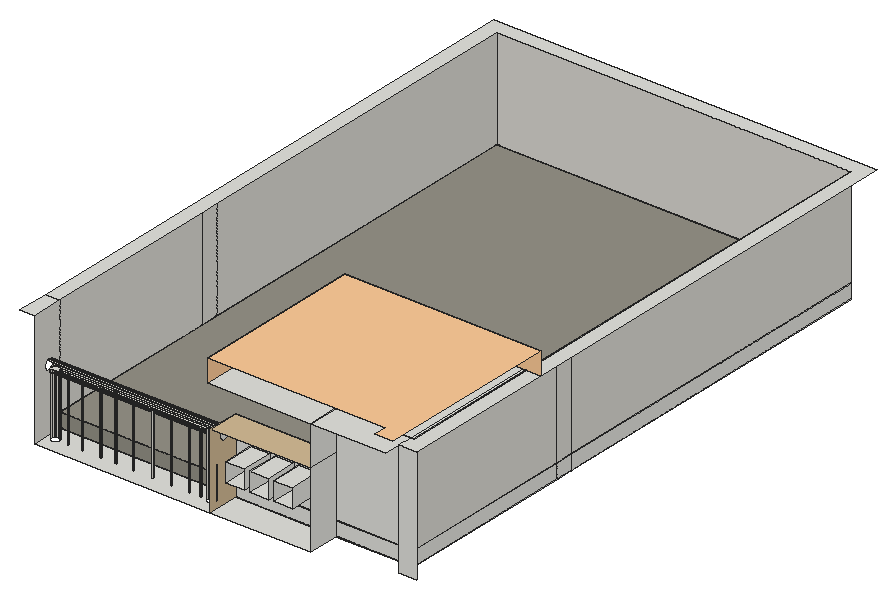
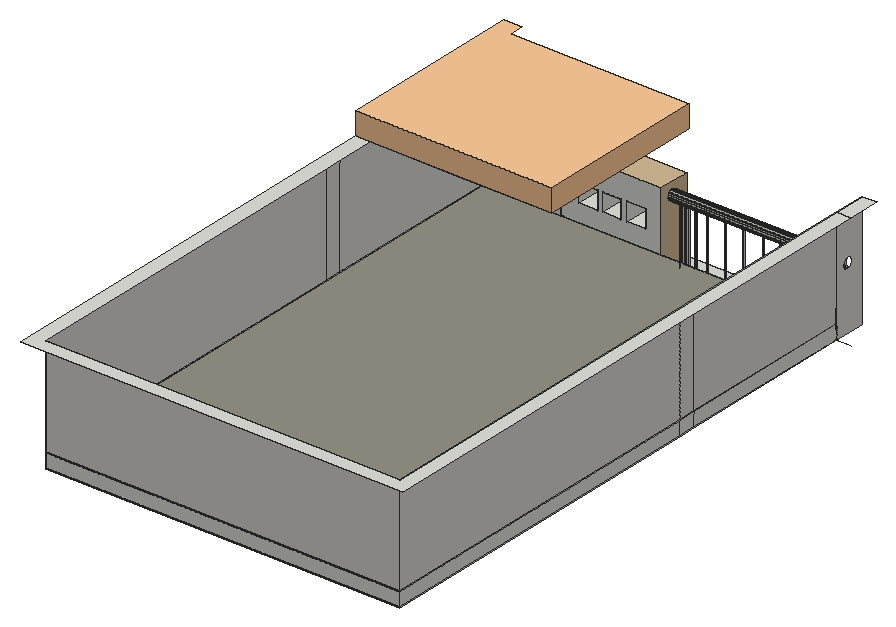
# SketchUp Ruby script. Lengths in inches.
U = 1.inch
M = Sketchup.active_model
def pt(a) = Geom::Point3d.new(a.map { |v| v * U })
def face(e, loops, mat)
  f = e.add_face(loops[0].map { |a| pt(a) })
  loops[1..].each { |l| e.add_face(l.map { |a| pt(a) }).erase! }
  f.material = f.back_material = mat if mat
  f
end
# faces: each face lists its corners as indices into pts; further lists are holes
def faces(e, pts, list, mat = nil) = list.each { |f| face(e, (f[0].is_a?(Array) ? f : [f]).map { |l| l.map { |i| pts[i] } }, mat) }
# xy, xz, yz: faces in a plane at the given z, y or x. An outline is a flat list of corners, or four numbers for a rectangle; further outlines are holes
def ring(l) = l.size == 4 ? [[l[0], l[1]], [l[2], l[1]], [l[2], l[3]], [l[0], l[3]]] : l.each_slice(2).to_a
def flat(e, list, mat, &to3) = list.each { |f| face(e, (f[0].is_a?(Array) ? f : [f]).map { |l| ring(l).map { |u, v| to3.(u, v) } }, mat) }
def xy(e, z, list, mat = nil) = flat(e, list, mat) { |x, y| [x, y, z] }
def xz(e, y, list, mat = nil) = flat(e, list, mat) { |x, z| [x, y, z] }
def yz(e, x, list, mat = nil) = flat(e, list, mat) { |y, z| [x, y, z] }
def lines(e, pts, list) = list.each { |a, b| e.add_line(pt(pts[a]), pt(pts[b])) }
# prism: a flat outline (further loops are holes) pulled along v
def prism(e, loops, v, mat = nil)
  f = face(e, loops, mat); d = Geom::Vector3d.new(v.map { |x| x * U })
  f.pushpull(f.normal.samedirection?(d) ? d.length : -d.length)
end
def box(e, o, s, mat = nil) = prism(e, [[o, [o[0] + s[0], o[1], o[2]], [o[0] + s[0], o[1] + s[1], o[2]], [o[0], o[1] + s[1], o[2]]]], [0, 0, s[2]], mat)
def at(x, y, z, deg = 0) = Geom::Transformation.translation(pt([x, y, z])) * Geom::Transformation.rotation(ORIGIN, Z_AXIS, deg.degrees)
def axes(o, x, y, z) = Geom::Transformation.new([*x, 0, *y, 0, *z, 0, *pt(o).to_a, 1])
def part(name) = M.definitions.add(name)
# library, detail: a bought-in or finely detailed component or shape, given as its bounding box
def library(name, o, s) = part(name).tap { |d| box(d.entities, o, s) }
def detail(e, o, s) = box(e.add_group.entities, o, s)
def put(e, d, t, mat = nil) = e.add_instance(d, t).tap { |i| i.material = mat if mat }
def group(e, t, mat = nil) = e.add_group.tap { |g| g.transformation = t; g.material = mat if mat }.entities
root = M.entities
M.materials.add("[Color C02]").color = [255, 204, 153]
M.materials.add("[Formica Beige]").color = [211, 187, 149]
M.materials.add("[Formica Graystone]").color = [149, 146, 135]
M.materials.add("[Terrazzo Tile Light]").color = [219, 217, 210]
xy(root,120,[[[9,41.58,119.1,61.39],[14.33,48.46,13.65,48.55,13.02,48.81,12.48,49.23,12.06,49.77,11.8,50.4,11.71,51.08,11.8,51.76,12.06,52.4,12.48,52.9375,13.02,53.36,13.65,53.62,14.33,53.71,15.01,53.62,15.64,53.36,16.1875,52.9375,16.6,52.4,16.87,51.76,16.96,51.08,16.87,50.4,16.6,49.77,16.1875,49.23,15.64,48.81,15.01,48.55],[112.21,48.46,111.53,48.55,110.89,48.81,110.35,49.23,109.93,49.77,109.67,50.4,109.58,51.08,109.67,51.76,109.93,52.4,110.35,52.9375,110.89,53.36,111.53,53.62,112.21,53.71,112.89,53.62,113.52,53.36,114.0625,52.9375,114.48,52.4,114.74,51.76,114.83,51.08,114.74,50.4,114.48,49.77,114.0625,49.23,113.52,48.81,112.89,48.55],[75.6,50.32,75.46,50.34,75.32,50.4,75.21,50.48,75.12,50.6,75.0625,50.74,75.04,50.88,75.0625,51.03,75.12,51.16,75.21,51.28,75.32,51.37,75.46,51.43,75.6,51.44,75.75,51.43,75.89,51.37,76,51.28,76.09,51.16,76.15,51.03,76.17,50.88,76.15,50.74,76.09,50.6,76,50.48,75.89,50.4,75.75,50.34],[31.29,50.32,31.15,50.34,31.01,50.4,30.89,50.48,30.8,50.6,30.75,50.74,30.73,50.88,30.75,51.03,30.8,51.16,30.89,51.28,31.01,51.37,31.15,51.43,31.29,51.44,31.4375,51.43,31.57,51.37,31.69,51.28,31.78,51.16,31.84,51.03,31.85,50.88,31.84,50.74,31.78,50.6,31.69,50.48,31.57,50.4,31.4375,50.34],[52.1,50.32,51.96,50.34,51.82,50.4,51.71,50.48,51.62,50.6,51.5625,50.74,51.54,50.88,51.5625,51.03,51.62,51.16,51.71,51.28,51.82,51.37,51.96,51.43,52.1,51.44,52.25,51.43,52.39,51.37,52.5,51.28,52.59,51.16,52.65,51.03,52.67,50.88,52.65,50.74,52.59,50.6,52.5,50.48,52.39,50.4,52.25,50.34],[63.23,50.32,63.08,50.34,62.95,50.4,62.83,50.48,62.74,50.6,62.6875,50.74,62.67,50.88,62.6875,51.03,62.74,51.16,62.83,51.28,62.95,51.37,63.08,51.43,63.23,51.44,63.375,51.43,63.51,51.37,63.63,51.28,63.72,51.16,63.77,51.03,63.79,50.88,63.77,50.74,63.72,50.6,63.63,50.48,63.51,50.4,63.375,50.34],[42.67,50.32,42.52,50.34,42.39,50.4,42.27,50.48,42.18,50.6,42.125,50.74,42.1,50.88,42.125,51.03,42.18,51.16,42.27,51.28,42.39,51.37,42.52,51.43,42.67,51.44,42.8125,51.43,42.95,51.37,43.06,51.28,43.15,51.16,43.21,51.03,43.23,50.88,43.21,50.74,43.15,50.6,43.06,50.48,42.95,50.4,42.8125,50.34],[87.1,50.32,86.96,50.34,86.82,50.4,86.71,50.48,86.62,50.6,86.5625,50.74,86.54,50.88,86.5625,51.03,86.62,51.16,86.71,51.28,86.82,51.37,86.96,51.43,87.1,51.44,87.25,51.43,87.39,51.37,87.5,51.28,87.59,51.16,87.65,51.03,87.67,50.88,87.65,50.74,87.59,50.6,87.5,50.48,87.39,50.4,87.25,50.34],[22.54,50.32,22.4,50.34,22.26,50.4,22.14,50.48,22.05,50.6,22,50.74,21.98,50.88,22,51.03,22.05,51.16,22.14,51.28,22.26,51.37,22.4,51.43,22.54,51.44,22.6875,51.43,22.82,51.37,22.94,51.28,23.03,51.16,23.09,51.03,23.1,50.88,23.09,50.74,23.03,50.6,22.94,50.48,22.82,50.4,22.6875,50.34],[105.42,50.32,105.27,50.34,105.14,50.4,105.02,50.48,104.93,50.6,104.875,50.74,104.85,50.88,104.875,51.03,104.93,51.16,105.02,51.28,105.14,51.37,105.27,51.43,105.42,51.44,105.5625,51.43,105.7,51.37,105.81,51.28,105.9,51.16,105.96,51.03,105.98,50.88,105.96,50.74,105.9,50.6,105.81,50.48,105.7,50.4,105.5625,50.34],[98.42,50.32,98.27,50.34,98.14,50.4,98.02,50.48,97.93,50.6,97.875,50.74,97.85,50.88,97.875,51.03,97.93,51.16,98.02,51.28,98.14,51.37,98.27,51.43,98.42,51.44,98.5625,51.43,98.7,51.37,98.81,51.28,98.9,51.16,98.96,51.03,98.98,50.88,98.96,50.74,98.9,50.6,98.81,50.48,98.7,50.4,98.5625,50.34]],[119.1,41.58,181.98,61.39],[9,61.39,231,172.96],[9,172.96,231,184.44],[9,184.44,231,403.39]])
xy(root,120.27,[[9,61.39,231,403.39]])
xy(root,129,[[9,61.39,231,403.39]])
xy(root,129.27,[[9,61.39,231,403.39]],"[Formica Graystone]")
xy(root,140.26,[[128.8125,41.58,140.5625,61.39],[144.125,41.58,155.875,61.39],[158.8125,41.58,170.5625,61.39]])
xy(root,152.01,[[128.8125,41.58,140.5625,61.39],[144.125,41.58,155.875,61.39],[158.8125,41.58,170.5625,61.39]])
xy(root,159.78,[[12.24,49.53,16.42,49.53,16.6,49.77,16.87,50.4,16.96,51.08,16.87,51.76,16.6,52.4,16.1875,52.9375,15.64,53.36,15.01,53.62,14.33,53.71,13.65,53.62,13.02,53.36,12.48,52.9375,12.06,52.4,11.8,51.76,11.71,51.08,11.8,50.4,12.06,49.77]])
xy(root,166.92,[[119.1,41.58,181.98,61.39]],"[Formica Beige]")
xy(root,192,[[0,41.58,9,61.39],[117.3125,41.58,181.98,149.14],[181.98,41.58,228.875,61.39],[228.875,52.39,240,52.39,240,149.14,231,149.14,231,61.39,228.875,61.39],[0,61.39,9,61.39,9,403.39,231,403.39,231,149.14,240,149.14,240,412.39,0,412.39],
  [181.98,61.39,228.875,149.14],[228.875,61.39,231,149.14]])
xy(root,206.25,[[228.875,33.14,240,33.14,240,149.14,117.3125,149.14,117.3125,41.58,228.875,41.58]],"[Color C02]")
xz(root,52.39,[[228.875,120,240,192]])
xz(root,61.39,[[9,120,119.1,120.27],[119.1,120,181.98,120.27],[181.98,120,231,120.27],[119.1,120.27,181.98,129],[181.98,120.27,231,129],
  [9,129,119.1,129.27],[119.1,129,181.98,129.27],[181.98,129,231,129.27],[[119.1,129.27,181.98,166.92],[128.8125,140.26,140.5625,152.01],[144.125,140.26,155.875,152.01],[158.8125,140.26,170.5625,152.01]],[181.98,129.27,231,192]])
xz(root,61.39,[[9,120.27,119.1,129]],"[Formica Graystone]")
xz(root,149.14,[[117.3125,192,240,206.25]],"[Color C02]")
xz(root,403.39,[[9,120,231,120.27],[9,120.27,231,129],[9,129,231,129.27]])
xz(root,403.39,[[9,129.27,231,192]],"[Terrazzo Tile Light]")
yz(root,9,[[61.39,120,172.96,120.27],[172.96,120,184.44,120.27],[184.44,120,403.39,120.27],[61.39,120.27,172.96,129],[172.96,120.27,184.44,129],
  [184.44,120.27,403.39,129],[61.39,129,172.96,129.27],[172.96,129,184.44,129.27],[184.44,129,403.39,129.27]])
yz(root,9,[[[41.58,120,61.39,192],[52.9,156.41,52.03,156.52,51.22,156.86,50.52,157.4,49.98,158.09,49.64,158.91,49.53,159.78,49.64,160.66,49.98,161.47,50.52,162.17,51.22,162.7,52.03,163.04,52.9,163.16,53.78,163.04,54.59,162.7,55.29,162.17,55.83,161.47,56.16,160.66,56.28,159.78,56.16,158.91,55.83,158.09,55.29,157.4,54.59,156.86,53.78,156.52]],[61.39,129.27,172.96,192],[172.96,129.27,184.44,192],[184.44,129.27,403.39,192]],"[Terrazzo Tile Light]")
yz(root,117.3125,[[41.58,192,149.14,206.25]],"[Color C02]")
yz(root,119.1,[[52.9,156.41,53.78,156.52,54.59,156.86,55.29,157.4,55.83,158.09,56.16,158.91,56.28,159.78,56.16,160.66,55.83,161.47,55.29,162.17,54.59,162.7,53.78,163.04,52.9,163.16,52.03,163.04,51.22,162.7,50.52,162.17,49.98,161.47,49.64,160.66,49.53,159.78,49.64,158.91,49.98,158.09,50.52,157.4,51.22,156.86,52.03,156.52]])
yz(root,119.1,[[[41.58,120,61.39,166.92],[52.9,156.41,53.78,156.52,54.59,156.86,55.29,157.4,55.83,158.09,56.16,158.91,56.28,159.78,56.16,160.66,55.83,161.47,55.29,162.17,54.59,162.7,53.78,163.04,52.9,163.16,52.03,163.04,51.22,162.7,50.52,162.17,49.98,161.47,49.64,160.66,49.53,159.78,49.64,158.91,49.98,158.09,50.52,157.4,51.22,156.86,52.03,156.52]]],"[Formica Beige]")
yz(root,128.8125,[[41.58,140.26,61.39,152.01]])
yz(root,140.5625,[[41.58,140.26,61.39,152.01]])
yz(root,144.125,[[41.58,140.26,61.39,152.01]])
yz(root,155.875,[[41.58,140.26,61.39,152.01]])
yz(root,158.8125,[[41.58,140.26,61.39,152.01]])
yz(root,170.5625,[[41.58,140.26,61.39,152.01]])
yz(root,181.98,[[41.58,120,61.39,166.92],[41.58,166.92,61.39,192]])
yz(root,231,[[61.39,120,172.96,120.27],[172.96,120,184.44,120.27],[184.44,120,403.39,120.27],[61.39,120.27,172.96,129],[172.96,120.27,184.44,129],
  [184.44,120.27,403.39,129],[61.39,129,172.96,129.27],[172.96,129,184.44,129.27],[184.44,129,403.39,129.27]])
yz(root,231,[[61.39,129.27,172.96,192],[172.96,129.27,184.44,192],[184.44,129.27,403.39,192]],"[Terrazzo Tile Light]")
p = [[42.18,51.16,120],[42.125,51.03,120],[42.125,51.03,159.4375],[42.18,51.16,159.4375],[43.21,51.03,120],[43.15,51.16,120],
  [43.15,51.16,159.4375],[43.21,51.03,159.4375],[51.62,51.16,120],[51.5625,51.03,120],[51.5625,51.03,160.66],[51.62,51.16,160.66],
  [52.65,51.03,120],[52.59,51.16,120],[52.59,51.16,160.66],[52.65,51.03,160.66],[62.74,51.16,120],[62.6875,51.03,120],
  [62.6875,51.03,158.09],[62.74,51.16,158.09],[63.77,51.03,120],[63.72,51.16,120],[63.72,51.16,158.09],[63.77,51.03,158.09],
  [75.12,51.16,120],[75.0625,51.03,120],[75.0625,51.03,157.625],[75.12,51.16,157.625],[76.15,51.03,120],[76.09,51.16,120],
  [76.09,51.16,157.625],[76.15,51.03,157.625],[86.62,51.16,120],[86.5625,51.03,120],[86.5625,51.03,158.1875],[86.62,51.16,158.1875],
  [87.65,51.03,120],[87.59,51.16,120],[87.59,51.16,158.1875],[87.65,51.03,158.1875],[97.93,51.16,120],[97.875,51.03,120],
  [97.875,51.03,157.5625],[97.93,51.16,157.5625],[98.96,51.03,120],[98.9,51.16,120],[98.9,51.16,157.5625],[98.96,51.03,157.5625],
  [104.93,51.16,120],[104.875,51.03,120],[104.875,51.03,157.8125],[104.93,51.16,157.8125],[105.96,51.03,120],[105.9,51.16,120],
  [105.9,51.16,157.8125],[105.96,51.03,157.8125],[11.8,51.76,120],[11.71,51.08,120],[11.71,51.08,159.78],[11.8,51.76,159.78],
  [16.96,51.08,120],[16.87,51.76,120],[16.87,51.76,159.78],[16.96,51.08,159.78],[109.67,51.76,120],[109.58,51.08,120],
  [109.58,51.08,159],[109.67,51.76,159],[114.83,51.08,120],[114.74,51.76,120],[114.74,51.76,159],[114.83,51.08,159],
  [22.14,51.28,120],[22.05,51.16,120],[22.05,51.16,159.5],[22.14,51.28,159.5],[23.03,51.16,120],[22.94,51.28,120],
  [22.94,51.28,159.5],[23.03,51.16,159.5],[30.89,51.28,120],[30.8,51.16,120],[30.8,51.16,159.875],[30.89,51.28,159.875],
  [31.78,51.16,120],[31.69,51.28,120],[31.69,51.28,159.875],[31.78,51.16,159.875],[42.27,51.28,120],[42.27,51.28,159.4375],
  [43.06,51.28,120],[43.06,51.28,159.4375],[51.71,51.28,120],[51.71,51.28,160.66],[52.5,51.28,120],[52.5,51.28,160.66],
  [62.83,51.28,120],[62.83,51.28,158.09],[63.63,51.28,120],[63.63,51.28,158.09],[75.21,51.28,120],[75.21,51.28,157.625],
  [76,51.28,120],[76,51.28,157.625],[86.71,51.28,120],[86.71,51.28,158.1875],[87.5,51.28,120],[87.5,51.28,158.1875],
  [98.02,51.28,120],[98.02,51.28,157.5625],[98.81,51.28,120],[98.81,51.28,157.5625],[105.02,51.28,120],[105.02,51.28,157.8125],
  [105.81,51.28,120],[105.81,51.28,157.8125],[22.26,51.37,120],[22.26,51.37,159.5],[22.82,51.37,120],[22.82,51.37,159.5],
  [31.01,51.37,120],[31.01,51.37,159.875],[31.57,51.37,120],[31.57,51.37,159.875],[42.39,51.37,120],[42.39,51.37,159.4375],
  [42.95,51.37,120],[42.95,51.37,159.4375],[51.82,51.37,120],[51.82,51.37,160.66],[52.39,51.37,120],[52.39,51.37,160.66],
  [62.95,51.37,120],[62.95,51.37,158.09],[63.51,51.37,120],[63.51,51.37,158.09],[75.32,51.37,120],[75.32,51.37,157.625],
  [75.89,51.37,120],[75.89,51.37,157.625],[86.82,51.37,120],[86.82,51.37,158.1875],[87.39,51.37,120],[87.39,51.37,158.1875],
  [98.14,51.37,120],[98.14,51.37,157.5625],[98.7,51.37,120],[98.7,51.37,157.5625],[105.14,51.37,120],[105.14,51.37,157.8125],
  [105.7,51.37,120],[105.7,51.37,157.8125],[22.4,51.43,120],[22.4,51.43,159.5],[22.54,51.44,120],[22.54,51.44,159.5],
  [22.6875,51.43,120],[22.6875,51.43,159.5],[31.15,51.43,120],[31.15,51.43,159.875],[31.29,51.44,120],[31.29,51.44,159.875],
  [31.4375,51.43,120],[31.4375,51.43,159.875],[42.52,51.43,120],[42.52,51.43,159.4375],[42.67,51.44,120],[42.67,51.44,159.4375],
  [42.8125,51.43,120],[42.8125,51.43,159.4375],[51.96,51.43,120],[51.96,51.43,160.66],[52.1,51.44,120],[52.1,51.44,160.66],
  [52.25,51.43,120],[52.25,51.43,160.66],[63.08,51.43,120],[63.08,51.43,158.09],[63.23,51.44,120],[63.23,51.44,158.09],
  [63.375,51.43,120],[63.375,51.43,158.09],[75.46,51.43,120],[75.46,51.43,157.625],[75.6,51.44,120],[75.6,51.44,157.625],
  [75.75,51.43,120],[75.75,51.43,157.625],[86.96,51.43,120],[86.96,51.43,158.1875],[87.1,51.44,120],[87.1,51.44,158.1875],
  [87.25,51.43,120],[87.25,51.43,158.1875],[98.27,51.43,120],[98.27,51.43,157.5625],[98.42,51.44,120],[98.42,51.44,157.5625],
  [98.5625,51.43,120],[98.5625,51.43,157.5625],[105.27,51.43,120],[105.27,51.43,157.8125],[105.42,51.44,120],[105.42,51.44,157.8125],
  [105.5625,51.43,120],[105.5625,51.43,157.8125],[12.06,52.4,120],[12.06,52.4,159.78],[16.6,52.4,120],[16.6,52.4,159.78],
  [109.93,52.4,120],[109.93,52.4,159],[114.48,52.4,120],[114.48,52.4,159],[12.48,52.9375,120],[12.48,52.9375,159.78],
  [16.1875,52.9375,120],[16.1875,52.9375,159.78],[110.35,52.9375,120],[110.35,52.9375,159],[114.0625,52.9375,120],[114.0625,52.9375,159],
  [13.02,53.36,120],[13.02,53.36,159.78],[15.64,53.36,120],[15.64,53.36,159.78],[110.89,53.36,120],[110.89,53.36,159],
  [113.52,53.36,120],[113.52,53.36,159],[13.65,53.62,120],[13.65,53.62,159.78],[15.01,53.62,120],[15.01,53.62,159.78],
  [111.53,53.62,120],[111.53,53.62,159],[112.89,53.62,120],[112.89,53.62,159],[14.33,53.71,120],[14.33,53.71,159.78],
  [112.21,53.71,120],[112.21,53.71,159],[119.1,52.9,156.41],[119.1,52.03,156.52],[9,52.03,156.52],[9,52.9,156.41],
  [119.1,53.78,156.52],[9,53.78,156.52],[119.1,51.22,156.86],[9,51.22,156.86],[119.1,54.59,156.86],[9,54.59,156.86],
  [119.1,55.29,157.4],[9,55.29,157.4],[119.1,55.83,158.09],[9,55.83,158.09],[119.1,56.16,158.91],[9,56.16,158.91],
  [119.1,56.28,159.78],[9,56.28,159.78],[119.1,56.16,160.66],[9,56.16,160.66],[119.1,55.83,161.47],[9,55.83,161.47],
  [119.1,55.29,162.17],[9,55.29,162.17],[119.1,54.59,162.7],[9,54.59,162.7],[119.1,51.22,162.7],[119.1,52.03,163.04],
  [9,52.03,163.04],[9,51.22,162.7],[119.1,53.78,163.04],[9,53.78,163.04],[119.1,52.9,163.16],[9,52.9,163.16],
  [9,61.39,120],[0,61.39,120]]
faces(root,p,[[0,1,2,3],[4,5,6,7],[8,9,10,11],[12,13,14,15],[16,17,18,19],[20,21,22,23],[24,25,26,27],[28,29,30,31],
  [32,33,34,35],[36,37,38,39],[40,41,42,43],[44,45,46,47],[48,49,50,51],[52,53,54,55],[56,57,58,59],[60,61,62,63],
  [64,65,66,67],[68,69,70,71],[72,73,74,75],[76,77,78,79],[80,81,82,83],[84,85,86,87],[88,0,3,89],[5,90,91,6],
  [92,8,11,93],[13,94,95,14],[96,16,19,97],[21,98,99,22],[100,24,27,101],[29,102,103,30],[104,32,35,105],[37,106,107,38],
  [108,40,43,109],[45,110,111,46],[112,48,51,113],[53,114,115,54],[116,72,75,117],[77,118,119,78],[120,80,83,121],[85,122,123,86],
  [124,88,89,125],[90,126,127,91],[128,92,93,129],[94,130,131,95],[132,96,97,133],[98,134,135,99],[136,100,101,137],[102,138,139,103],
  [140,104,105,141],[106,142,143,107],[144,108,109,145],[110,146,147,111],[148,112,113,149],[114,150,151,115],[152,116,117,153],[154,152,153,155],
  [156,154,155,157],[118,156,157,119],[158,120,121,159],[160,158,159,161],[162,160,161,163],[122,162,163,123],[164,124,125,165],[166,164,165,167],
  [168,166,167,169],[126,168,169,127],[170,128,129,171],[172,170,171,173],[174,172,173,175],[130,174,175,131],[176,132,133,177],[178,176,177,179],
  [180,178,179,181],[134,180,181,135],[182,136,137,183],[184,182,183,185],[186,184,185,187],[138,186,187,139],[188,140,141,189],[190,188,189,191],
  [192,190,191,193],[142,192,193,143],[194,144,145,195],[196,194,195,197],[198,196,197,199],[146,198,199,147],[200,148,149,201],[202,200,201,203],
  [204,202,203,205],[150,204,205,151],[206,56,59,207],[61,208,209,62],[210,64,67,211],[69,212,213,70],[214,206,207,215],[208,216,217,209],
  [218,210,211,219],[212,220,221,213],[222,214,215,223],[216,224,225,217],[226,218,219,227],[220,228,229,221],[230,222,223,231],[224,232,233,225],
  [234,226,227,235],[228,236,237,229],[238,230,231,239],[232,238,239,233],[240,234,235,241],[236,240,241,237],[242,243,244,245],[246,242,245,247],
  [243,248,249,244],[250,246,247,251],[252,250,251,253],[254,252,253,255],[256,254,255,257],[258,256,257,259],[260,258,259,261],[262,260,261,263],
  [264,262,263,265],[266,264,265,267],[268,269,270,271],[272,266,267,273],[269,274,275,270],[274,272,273,275]],"[Terrazzo Tile Light]")
lines(root,p,[[276,277]])
